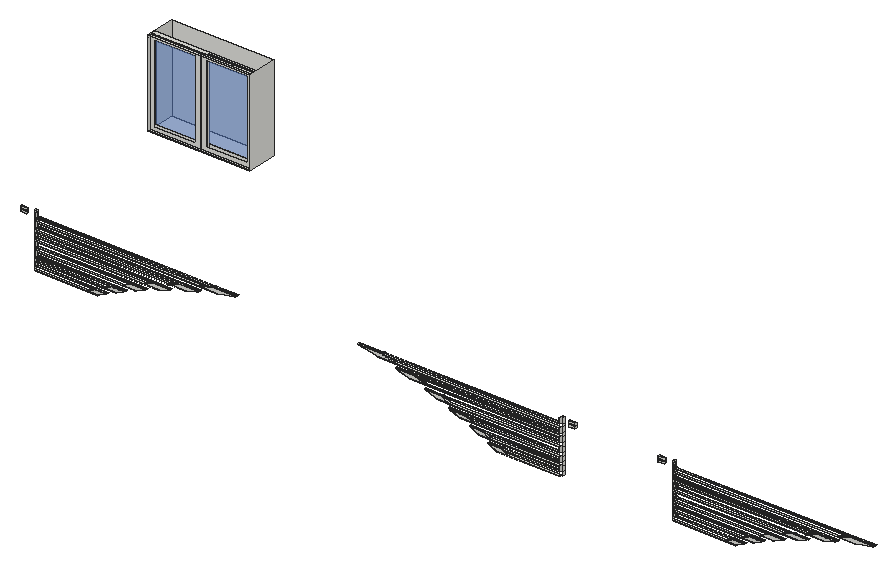
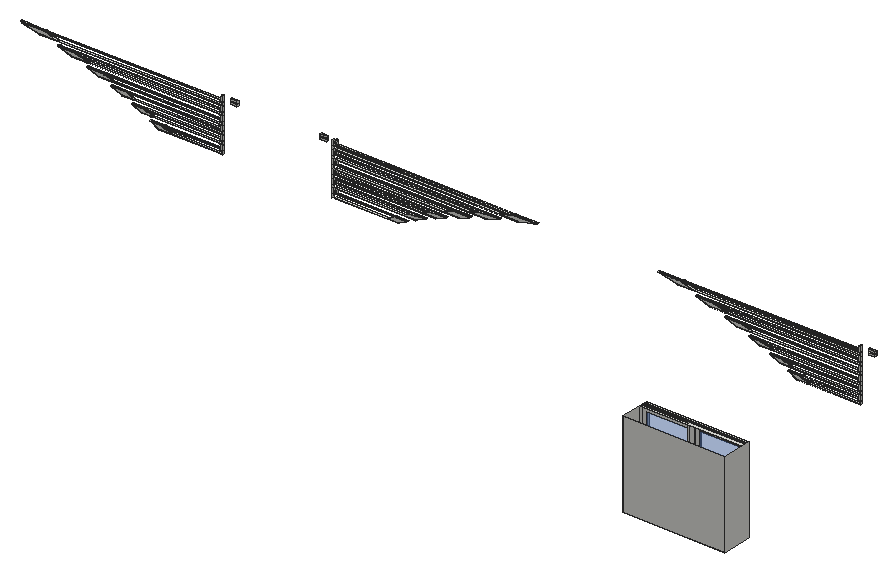
# SketchUp Ruby script. Lengths in inches.
U = 1.inch
M = Sketchup.active_model
def pt(a) = Geom::Point3d.new(a.map { |v| v * U })
def face(e, loops, mat)
  f = e.add_face(loops[0].map { |a| pt(a) })
  loops[1..].each { |l| e.add_face(l.map { |a| pt(a) }).erase! }
  f.material = f.back_material = mat if mat
  f
end
# faces: each face lists its corners as indices into pts; further lists are holes
def faces(e, pts, list, mat = nil) = list.each { |f| face(e, (f[0].is_a?(Array) ? f : [f]).map { |l| l.map { |i| pts[i] } }, mat) }
# xy, xz, yz: faces in a plane at the given z, y or x. An outline is a flat list of corners, or four numbers for a rectangle; further outlines are holes
def ring(l) = l.size == 4 ? [[l[0], l[1]], [l[2], l[1]], [l[2], l[3]], [l[0], l[3]]] : l.each_slice(2).to_a
def flat(e, list, mat, &to3) = list.each { |f| face(e, (f[0].is_a?(Array) ? f : [f]).map { |l| ring(l).map { |u, v| to3.(u, v) } }, mat) }
def xy(e, z, list, mat = nil) = flat(e, list, mat) { |x, y| [x, y, z] }
def xz(e, y, list, mat = nil) = flat(e, list, mat) { |x, z| [x, y, z] }
def yz(e, x, list, mat = nil) = flat(e, list, mat) { |y, z| [x, y, z] }
def lines(e, pts, list) = list.each { |a, b| e.add_line(pt(pts[a]), pt(pts[b])) }
# prism: a flat outline (further loops are holes) pulled along v
def prism(e, loops, v, mat = nil)
  f = face(e, loops, mat); d = Geom::Vector3d.new(v.map { |x| x * U })
  f.pushpull(f.normal.samedirection?(d) ? d.length : -d.length)
end
def box(e, o, s, mat = nil) = prism(e, [[o, [o[0] + s[0], o[1], o[2]], [o[0] + s[0], o[1] + s[1], o[2]], [o[0], o[1] + s[1], o[2]]]], [0, 0, s[2]], mat)
def at(x, y, z, deg = 0) = Geom::Transformation.translation(pt([x, y, z])) * Geom::Transformation.rotation(ORIGIN, Z_AXIS, deg.degrees)
def axes(o, x, y, z) = Geom::Transformation.new([*x, 0, *y, 0, *z, 0, *pt(o).to_a, 1])
def part(name) = M.definitions.add(name)
# library, detail: a bought-in or finely detailed component or shape, given as its bounding box
def library(name, o, s) = part(name).tap { |d| box(d.entities, o, s) }
def detail(e, o, s) = box(e.add_group.entities, o, s)
def put(e, d, t, mat = nil) = e.add_instance(d, t).tap { |i| i.material = mat if mat }
def group(e, t, mat = nil) = e.add_group.tap { |g| g.transformation = t; g.material = mat if mat }.entities
root = M.entities
M.materials.add("[Translucent Glass Blue]").color = [100, 149, 237]
M.materials["[Translucent Glass Blue]"].alpha = 0.5
c1 = part("Janela aluminio")
xy(c1.entities,0,[[0,0,47.24,1.57],[23.62,1.57,47.24,2.76],[0,2.76,25.98,3.9375],[0,3.9375,47.24,5.91]])
xy(c1.entities,43.31,[[0,0,47.24,1.57],[23.62,1.57,47.24,2.76],[0,2.76,0,5.91,47.24,5.91,47.24,3.9375,25.98,3.9375,25.98,2.76],[25.98,2.76,47.24,3.9375]])
xz(c1.entities,1.57,[[0,0,23.62,0,23.62,41.34,21.26,41.34,21.26,1.97,1.97,1.97,1.97,41.34,23.62,41.34,23.62,43.31,0,43.31],[[23.62,0,47.24,43.31],[25.7,1.97,45.28,41.34]]])
xz(c1.entities,2.76,[[[0,0,23.62,43.31],[2.36,2.36,21.26,40.94]],[23.62,0,25.98,43.31]])
xz(c1.entities,2.76,[[2.36,2.36,21.26,40.94]],"[Translucent Glass Blue]")
xz(c1.entities,3.9375,[[25.98,0,25.98,2.36,44.88,2.36,44.88,40.94,25.98,40.94,25.98,43.31,47.24,43.31,47.24,0]])
xz(c1.entities,3.9375,[[25.98,2.36,44.88,40.94]],"[Translucent Glass Blue]")
yz(c1.entities,0,[[0,0,1.57,43.31],[2.76,0,5.91,43.31]])
yz(c1.entities,23.62,[[1.57,0,2.76,43.31]])
yz(c1.entities,25.98,[[2.76,0,3.9375,43.31]])
yz(c1.entities,47.24,[[0,0,1.57,43.31],[1.57,0,2.76,43.31],[3.9375,0,5.91,43.31]])
xy(root,27.6875,[[193.54,12.93,230.17,13.56],[230.17,12.93,237.375,13.56],[518.74,12.93,525.9375,13.56],[525.9375,12.93,562.58,13.56],[643.44,12.93,680.08,13.56],
  [680.08,12.93,687.28,13.56],[193.54,13.81,230.17,14.31],[230.17,13.81,237.375,14.31],[518.74,13.81,525.9375,14.31],[525.9375,13.81,562.58,14.31],
  [643.44,13.81,680.08,14.31],[680.08,13.81,687.28,14.31]])
xy(root,28.18,[[192.75,12.93,230.17,14.31],[230.17,12.93,238.16,14.31],[517.95,12.93,525.9375,14.31],[525.9375,12.93,563.36,14.31],[642.65,12.93,680.08,14.31],
  [680.08,12.93,688.07,14.31]])
xy(root,29.54,[[145.1,172.4375,217.17,193.125]])
xy(root,30.61,[[192.75,12.93,234.88,14.31],[234.88,12.93,242.875,14.31],[513.24,12.93,521.23,14.31],[521.23,12.93,563.36,14.31],[642.65,12.93,684.79,14.31],
  [684.79,12.93,692.78,14.31]])
xy(root,31.1,[[193.54,12.93,234.88,13.56],[234.88,12.93,243.66,13.56],[512.45,12.93,521.23,13.56],[521.23,12.93,562.58,13.56],[643.44,12.93,684.79,13.56],
  [684.79,12.93,693.57,13.56],[193.54,13.81,234.88,14.31],[234.88,13.81,243.66,14.31],[512.45,13.81,521.23,14.31],[521.23,13.81,562.58,14.31],
  [643.44,13.81,684.79,14.31],[684.79,13.81,693.57,14.31]])
xy(root,33.81,[[193.54,12.93,242.07,13.56],[242.07,12.93,249.79,13.56],[506.32,12.93,514.05,13.56],[514.05,12.93,562.58,13.56],[643.44,12.93,691.97,13.56],
  [691.97,12.93,699.7,13.56],[193.54,13.81,242.07,14.31],[242.07,13.81,249.79,14.31],[506.32,13.81,514.05,14.31],[514.05,13.81,562.58,14.31],
  [643.44,13.81,691.97,14.31],[691.97,13.81,699.7,14.31]])
xy(root,34.3,[[192.75,12.93,242.07,14.31],[242.07,12.93,250.58,14.31],[505.53,12.93,514.05,14.31],[514.05,12.93,563.36,14.31],[642.65,12.93,691.97,14.31],
  [691.97,12.93,700.48,14.31]])
xy(root,36.73,[[192.75,12.93,247.27,14.31],[247.27,12.93,255.92,14.31],[500.19,12.93,508.84,14.31],[508.84,12.93,563.36,14.31],[642.65,12.93,697.18,14.31],
  [697.18,12.93,705.83,14.31]])
xy(root,37.22,[[193.54,12.93,247.27,13.56],[247.27,12.93,256.71,13.56],[499.4,12.93,508.84,13.56],[508.84,12.93,562.58,13.56],[643.44,12.93,697.18,13.56],
  [697.18,12.93,706.61,13.56],[193.54,13.81,247.27,14.31],[247.27,13.81,256.71,14.31],[499.4,13.81,508.84,14.31],[508.84,13.81,562.58,14.31],
  [643.44,13.81,697.18,14.31],[697.18,13.81,706.61,14.31]])
xy(root,39.93,[[193.54,12.93,255.42,13.56],[255.42,12.93,263.81,13.56],[492.31,12.93,500.7,13.56],[500.7,12.93,562.58,13.56],[643.44,12.93,705.32,13.56],
  [705.32,12.93,713.71,13.56],[193.54,13.81,255.42,14.31],[255.42,13.81,263.81,14.31],[492.31,13.81,500.7,14.31],[500.7,13.81,562.58,14.31],
  [643.44,13.81,705.32,14.31],[705.32,13.81,713.71,14.31]])
xy(root,40.42,[[192.75,12.93,255.42,14.31],[255.42,12.93,264.59,14.31],[491.52,12.93,500.7,14.31],[500.7,12.93,563.36,14.31],[642.65,12.93,705.32,14.31],
  [705.32,12.93,714.5,14.31]])
xy(root,42.85,[[192.75,12.93,261.22,14.31],[261.22,12.93,270.68,14.31],[485.43,12.93,494.89,14.31],[494.89,12.93,563.36,14.31],[642.65,12.93,711.13,14.31],
  [711.13,12.93,720.59,14.31]])
xy(root,43.34,[[193.54,12.93,261.22,13.56],[261.22,12.93,271.47,13.56],[484.64,12.93,494.89,13.56],[494.89,12.93,562.58,13.56],[643.44,12.93,711.13,13.56],
  [711.13,12.93,721.38,13.56],[193.54,13.81,261.22,14.31],[261.22,13.81,271.47,14.31],[484.64,13.81,494.89,14.31],[494.89,13.81,562.58,14.31],
  [643.44,13.81,711.13,14.31],[711.13,13.81,721.38,14.31]])
xy(root,46.05,[[193.54,12.93,270.51,13.56],[270.51,12.93,279.92,13.56],[476.19,12.93,485.61,13.56],[485.61,12.93,562.58,13.56],[643.44,12.93,720.41,13.56],
  [720.41,12.93,729.83,13.56],[193.54,13.81,270.51,14.31],[270.51,13.81,279.92,14.31],[476.19,13.81,485.61,14.31],[485.61,13.81,562.58,14.31],
  [643.44,13.81,720.41,14.31],[720.41,13.81,729.83,14.31]])
xy(root,46.54,[[192.75,12.93,270.51,14.31],[270.51,12.93,280.71,14.31],[475.4,12.93,485.61,14.31],[485.61,12.93,563.36,14.31],[642.65,12.93,720.41,14.31],
  [720.41,12.93,730.62,14.31]])
xy(root,48.97,[[192.75,12.93,277.22,14.31],[277.22,12.93,287.71,14.31],[468.41,12.93,478.89,14.31],[478.89,12.93,563.36,14.31],[642.65,12.93,727.13,14.31],
  [727.13,12.93,737.61,14.31]])
xy(root,49.46,[[193.54,12.93,277.22,13.56],[277.22,12.93,288.49,13.56],[467.62,12.93,478.89,13.56],[478.89,12.93,562.58,13.56],[643.44,12.93,727.13,13.56],
  [727.13,12.93,738.4,13.56],[193.54,13.81,277.22,14.31],[277.22,13.81,288.49,14.31],[467.62,13.81,478.89,14.31],[478.89,13.81,562.58,14.31],
  [643.44,13.81,727.13,14.31],[727.13,13.81,738.4,14.31]])
xy(root,52.17,[[193.54,12.93,287.89,13.56],[287.89,12.93,298.9,13.56],[457.21,12.93,468.22,13.56],[468.22,12.93,562.58,13.56],[643.44,12.93,737.8,13.56],
  [737.8,12.93,748.81,13.56],[193.54,13.81,287.89,14.31],[287.89,13.81,298.9,14.31],[457.21,13.81,468.22,14.31],[468.22,13.81,562.58,14.31],
  [643.44,13.81,737.8,14.31],[737.8,13.81,748.81,14.31]])
xy(root,52.67,[[192.75,12.93,287.89,14.31],[287.89,12.93,299.6875,14.31],[456.42,12.93,468.22,14.31],[468.22,12.93,563.36,14.31],[642.65,12.93,737.8,14.31],
  [737.8,12.93,749.6,14.31]])
xy(root,55.09,[[192.75,12.93,296.02,14.31],[296.02,12.93,308.16,14.31],[447.95,12.93,460.1,14.31],[460.1,12.93,563.36,14.31],[642.65,12.93,745.92,14.31],
  [745.92,12.93,758.07,14.31]])
xy(root,55.59,[[193.54,12.93,296.02,13.56],[296.02,12.93,308.95,13.56],[447.17,12.93,460.1,13.56],[460.1,12.93,562.58,13.56],[643.44,12.93,745.92,13.56],
  [745.92,12.93,758.85,13.56],[193.54,13.81,296.02,14.31],[296.02,13.81,308.95,14.31],[447.17,13.81,460.1,14.31],[460.1,13.81,562.58,14.31],
  [643.44,13.81,745.92,14.31],[745.92,13.81,758.85,14.31]])
xy(root,58.29,[[193.54,12.93,309.22,13.56],[309.22,12.93,321.26,13.56],[434.85,12.93,446.9,13.56],[446.9,12.93,562.58,13.56],[643.44,12.93,759.12,13.56],
  [759.12,12.93,771.16,13.56],[193.54,13.81,309.22,14.31],[309.22,13.81,321.26,14.31],[434.85,13.81,446.9,14.31],[446.9,13.81,562.58,14.31],
  [643.44,13.81,759.12,14.31],[759.12,13.81,771.16,14.31]])
xy(root,58.79,[[192.75,12.93,309.22,14.31],[446.9,12.93,563.36,14.31],[642.65,12.93,759.12,14.31]])
xy(root,61.21,[[192.75,12.93,318.8,14.31],[318.8,12.93,334.49,14.31],[421.62,12.93,437.31,14.31],[437.31,12.93,563.36,14.31],[642.65,12.93,768.71,14.31],
  [768.71,12.93,784.4,14.31]])
xy(root,61.46,[[182.38,13.24,186.86,14.43],[569.26,13.24,573.73,14.43],[632.29,13.24,636.76,14.43]])
xy(root,61.71,[[193.54,12.93,318.8,13.56],[318.8,12.93,335.28,13.56],[420.83,12.93,437.31,13.56],[437.31,12.93,562.58,13.56],[643.44,12.93,768.71,13.56],
  [768.71,12.93,785.19,13.56],[193.54,13.81,318.8,14.31],[318.8,13.81,335.28,14.31],[420.83,13.81,437.31,14.31],[437.31,13.81,562.58,14.31],
  [643.44,13.81,768.71,14.31],[768.71,13.81,785.19,14.31]])
xy(root,62.75,[[182.38,13.24,186.86,14.43],[569.26,13.24,573.73,14.43],[632.29,13.24,636.76,14.43]])
xy(root,63.67,[[182.38,13.24,186.86,14.43],[569.26,13.24,573.73,14.43],[632.29,13.24,636.76,14.43]])
xz(root,12.93,[[230.17,28.18,238.16,28.18,242.875,30.61,234.88,30.61],[517.95,28.18,513.24,30.61,521.23,30.61,525.9375,28.18],[680.08,28.18,688.07,28.18,692.78,30.61,684.79,30.61],[242.07,34.3,250.58,34.3,255.92,36.73,247.27,36.73,243.08,34.82],[505.53,34.3,500.19,36.73,508.84,36.73,513.03,34.82,514.05,34.3],
  [691.97,34.3,700.48,34.3,705.83,36.73,697.18,36.73,692.98,34.82],[255.42,40.42,264.59,40.42,270.68,42.85,261.22,42.85,257.42,41.34],[491.52,40.42,485.43,42.85,494.89,42.85,498.6875,41.34,500.7,40.42],[705.32,40.42,714.5,40.42,720.59,42.85,711.13,42.85,707.33,41.34],[270.51,46.54,280.71,46.54,287.71,48.97,277.22,48.97,272.375,47.29],
  [475.4,46.54,468.41,48.97,478.89,48.97,483.74,47.29,485.61,46.54],[720.41,46.54,730.62,46.54,737.61,48.97,727.13,48.97,722.28,47.29],[287.89,52.67,299.6875,52.67,305.91,54.52,308.16,55.09,296.02,55.09],[456.42,52.67,450.21,54.52,447.95,55.09,460.1,55.09,468.22,52.67],[737.8,52.67,749.6,52.67,755.8125,54.52,758.07,55.09,745.92,55.09],
  [322.05,58.6,322.92,58.79,334.49,61.21,318.8,61.21,309.22,58.79,322.05,58.79],[434.07,58.6,433.19,58.79,421.62,61.21,437.31,61.21,446.9,58.79,434.07,58.79],[771.95,58.6,772.83,58.79,784.4,61.21,768.71,61.21,759.12,58.79,771.95,58.79]])
xz(root,13.24,[[182.38,61.46,186.86,62.75],[569.26,61.46,573.73,62.75],[632.29,61.46,636.76,62.75],[182.38,63.67,186.86,64.96],[569.26,63.67,573.73,64.96],
  [632.29,63.67,636.76,64.96]])
xz(root,14.31,[[230.17,28.18,234.88,30.61,242.875,30.61,238.16,28.18],[517.95,28.18,525.9375,28.18,521.23,30.61,513.24,30.61],[680.08,28.18,684.79,30.61,692.78,30.61,688.07,28.18],[242.07,34.3,243.08,34.82,247.27,36.73,255.92,36.73,250.58,34.3],[505.53,34.3,514.05,34.3,513.03,34.82,508.84,36.73,500.19,36.73],
  [691.97,34.3,692.98,34.82,697.18,36.73,705.83,36.73,700.48,34.3],[255.42,40.42,257.42,41.34,261.22,42.85,270.68,42.85,264.59,40.42],[491.52,40.42,500.7,40.42,498.6875,41.34,494.89,42.85,485.43,42.85],[705.32,40.42,707.33,41.34,711.13,42.85,720.59,42.85,714.5,40.42],[270.51,46.54,272.375,47.29,277.22,48.97,287.71,48.97,280.71,46.54],
  [475.4,46.54,485.61,46.54,483.74,47.29,478.89,48.97,468.41,48.97],[720.41,46.54,722.28,47.29,727.13,48.97,737.61,48.97,730.62,46.54],[287.89,52.67,296.02,55.09,308.16,55.09,305.91,54.52,299.6875,52.67],[456.42,52.67,468.22,52.67,460.1,55.09,447.95,55.09,450.21,54.52],[737.8,52.67,745.92,55.09,758.07,55.09,755.8125,54.52,749.6,52.67],
  [322.05,58.6,322.05,58.79,309.22,58.79,318.8,61.21,334.49,61.21,322.92,58.79],[434.07,58.6,434.07,58.79,446.9,58.79,437.31,61.21,421.62,61.21,433.19,58.79],[771.95,58.6,771.95,58.79,759.12,58.79,768.71,61.21,784.4,61.21,772.83,58.79]])
xz(root,14.43,[[182.38,61.46,186.86,62.75],[569.26,61.46,573.73,62.75],[632.29,61.46,636.76,62.75],[182.38,63.67,186.86,64.96],[569.26,63.67,573.73,64.96],
  [632.29,63.67,636.76,64.96]])
xz(root,193.125,[[145.1,29.54,217.17,90.15]])
yz(root,145.1,[[172.4375,29.54,193.125,90.15]])
yz(root,182.38,[[13.24,61.46,14.43,62.75],[13.24,63.67,14.43,64.96]])
yz(root,191.63,[[14.12,28.18,15.56,30.61],[14.12,30.61,15.56,34.3],[14.12,34.3,15.56,36.73],[14.12,36.73,15.56,40.42],[14.12,40.42,15.56,42.85],
  [14.12,42.85,15.56,46.54],[14.12,46.54,15.56,48.97],[14.12,48.97,15.56,52.67],[14.12,52.67,15.56,55.09],[14.12,55.09,15.56,58.79],
  [14.12,58.79,15.56,61.21],[14.12,61.21,15.56,64.91]])
yz(root,192.75,[[12.93,30.61,14.31,34.3],[14.31,30.61,15.56,34.3],[12.93,36.73,14.31,40.42],[14.31,36.73,15.56,40.42],[12.93,42.85,14.31,46.54],
  [14.31,42.85,15.56,46.54],[12.93,48.97,14.31,52.67],[14.31,48.97,15.56,52.67],[12.93,55.09,14.31,58.79],[14.31,55.09,15.56,58.79],
  [12.93,61.21,14.31,64.91],[14.31,61.21,15.56,64.91]])
yz(root,193.54,[[12.93,31.1,13.56,33.81],[13.81,31.1,14.31,33.81],[12.93,37.22,13.56,39.93],[13.81,37.22,14.31,39.93],[12.93,43.34,13.56,46.05],
  [13.81,43.34,14.31,46.05],[12.93,49.46,13.56,52.17],[13.81,49.46,14.31,52.17],[12.93,55.59,13.56,58.29],[13.81,55.59,14.31,58.29],
  [12.93,61.71,13.56,64.41],[13.81,61.71,14.31,64.41]])
yz(root,217.17,[[172.4375,29.54,193.125,90.15]])
yz(root,562.58,[[12.93,31.1,13.56,33.81],[13.81,31.1,14.31,33.81],[12.93,37.22,13.56,39.93],[13.81,37.22,14.31,39.93],[12.93,43.34,13.56,46.05],
  [13.81,43.34,14.31,46.05],[12.93,49.46,13.56,52.17],[13.81,49.46,14.31,52.17],[12.93,55.59,13.56,58.29],[13.81,55.59,14.31,58.29],
  [12.93,61.71,13.56,64.41],[13.81,61.71,14.31,64.41]])
yz(root,563.36,[[12.93,30.61,14.31,34.3],[14.31,30.61,15.56,34.3],[12.93,36.73,14.31,40.42],[14.31,36.73,15.56,40.42],[12.93,42.85,14.31,46.54],
  [14.31,42.85,15.56,46.54],[12.93,48.97,14.31,52.67],[14.31,48.97,15.56,52.67],[12.93,55.09,14.31,58.79],[14.31,55.09,15.56,58.79],
  [12.93,61.21,14.31,64.91],[14.31,61.21,15.56,64.91]])
yz(root,564.48,[[14.12,28.18,15.56,30.61],[14.12,30.61,15.56,34.3],[14.12,34.3,15.56,36.73],[14.12,36.73,15.56,40.42],[14.12,40.42,15.56,42.85],
  [14.12,42.85,15.56,46.54],[14.12,46.54,15.56,48.97],[14.12,48.97,15.56,52.67],[14.12,52.67,15.56,55.09],[14.12,55.09,15.56,58.79],
  [14.12,58.79,15.56,61.21],[14.12,61.21,15.56,64.91]])
yz(root,573.73,[[13.24,61.46,14.43,62.75],[13.24,63.67,14.43,64.96]])
yz(root,632.29,[[13.24,61.46,14.43,62.75],[13.24,63.67,14.43,64.96]])
yz(root,641.54,[[14.12,28.18,15.56,30.61],[14.12,30.61,15.56,34.3],[14.12,34.3,15.56,36.73],[14.12,36.73,15.56,40.42],[14.12,40.42,15.56,42.85],
  [14.12,42.85,15.56,46.54],[14.12,46.54,15.56,48.97],[14.12,48.97,15.56,52.67],[14.12,52.67,15.56,55.09],[14.12,55.09,15.56,58.79],
  [14.12,58.79,15.56,61.21],[14.12,61.21,15.56,64.91]])
yz(root,642.65,[[12.93,30.61,14.31,34.3],[14.31,30.61,15.56,34.3],[12.93,36.73,14.31,40.42],[14.31,36.73,15.56,40.42],[12.93,42.85,14.31,46.54],
  [14.31,42.85,15.56,46.54],[12.93,48.97,14.31,52.67],[14.31,48.97,15.56,52.67],[12.93,55.09,14.31,58.79],[14.31,55.09,15.56,58.79],
  [12.93,61.21,14.31,64.91],[14.31,61.21,15.56,64.91]])
yz(root,643.44,[[12.93,31.1,13.56,33.81],[13.81,31.1,14.31,33.81],[12.93,37.22,13.56,39.93],[13.81,37.22,14.31,39.93],[12.93,43.34,13.56,46.05],
  [13.81,43.34,14.31,46.05],[12.93,49.46,13.56,52.17],[13.81,49.46,14.31,52.17],[12.93,55.59,13.56,58.29],[13.81,55.59,14.31,58.29],
  [12.93,61.71,13.56,64.41],[13.81,61.71,14.31,64.41]])
p = [[234.88,14.31,30.61],[230.17,14.31,28.18],[230.17,12.93,28.18],[234.88,12.93,30.61],[238.16,14.31,28.18],[242.875,14.31,30.61],
  [242.875,12.93,30.61],[238.16,12.93,28.18],[517.95,14.31,28.18],[513.24,14.31,30.61],[513.24,12.93,30.61],[517.95,12.93,28.18],
  [521.23,14.31,30.61],[525.9375,14.31,28.18],[525.9375,12.93,28.18],[521.23,12.93,30.61],[684.79,14.31,30.61],[680.08,14.31,28.18],
  [680.08,12.93,28.18],[684.79,12.93,30.61],[688.07,14.31,28.18],[692.78,14.31,30.61],[692.78,12.93,30.61],[688.07,12.93,28.18],
  [243.08,14.31,34.82],[242.07,14.31,34.3],[242.07,12.93,34.3],[243.08,12.93,34.82],[250.58,14.31,34.3],[255.92,14.31,36.73],
  [255.92,12.93,36.73],[250.58,12.93,34.3],[505.53,14.31,34.3],[500.19,14.31,36.73],[500.19,12.93,36.73],[505.53,12.93,34.3],
  [513.03,14.31,34.82],[514.05,14.31,34.3],[514.05,12.93,34.3],[513.03,12.93,34.82],[692.98,14.31,34.82],[691.97,14.31,34.3],
  [691.97,12.93,34.3],[692.98,12.93,34.82],[700.48,14.31,34.3],[705.83,14.31,36.73],[705.83,12.93,36.73],[700.48,12.93,34.3],
  [247.27,14.31,36.73],[247.27,12.93,36.73],[508.84,14.31,36.73],[508.84,12.93,36.73],[697.18,14.31,36.73],[697.18,12.93,36.73],
  [257.42,14.31,41.34],[255.42,14.31,40.42],[255.42,12.93,40.42],[257.42,12.93,41.34],[264.59,14.31,40.42],[270.68,14.31,42.85],
  [270.68,12.93,42.85],[264.59,12.93,40.42],[491.52,14.31,40.42],[485.43,14.31,42.85],[485.43,12.93,42.85],[491.52,12.93,40.42],
  [498.6875,14.31,41.34],[500.7,14.31,40.42],[500.7,12.93,40.42],[498.6875,12.93,41.34],[707.33,14.31,41.34],[705.32,14.31,40.42],
  [705.32,12.93,40.42],[707.33,12.93,41.34],[714.5,14.31,40.42],[720.59,14.31,42.85],[720.59,12.93,42.85],[714.5,12.93,40.42],
  [261.22,14.31,42.85],[261.22,12.93,42.85],[494.89,14.31,42.85],[494.89,12.93,42.85],[711.13,14.31,42.85],[711.13,12.93,42.85],
  [272.375,14.31,47.29],[270.51,14.31,46.54],[270.51,12.93,46.54],[272.375,12.93,47.29],[280.71,14.31,46.54],[287.71,14.31,48.97],
  [287.71,12.93,48.97],[280.71,12.93,46.54],[475.4,14.31,46.54],[468.41,14.31,48.97],[468.41,12.93,48.97],[475.4,12.93,46.54],
  [483.74,14.31,47.29],[485.61,14.31,46.54],[485.61,12.93,46.54],[483.74,12.93,47.29],[722.28,14.31,47.29],[720.41,14.31,46.54],
  [720.41,12.93,46.54],[722.28,12.93,47.29],[730.62,14.31,46.54],[737.61,14.31,48.97],[737.61,12.93,48.97],[730.62,12.93,46.54],
  [277.22,14.31,48.97],[277.22,12.93,48.97],[478.89,14.31,48.97],[478.89,12.93,48.97],[727.13,14.31,48.97],[727.13,12.93,48.97],
  [296.02,14.31,55.09],[287.89,14.31,52.67],[287.89,12.93,52.67],[296.02,12.93,55.09],[299.6875,14.31,52.67],[305.91,14.31,54.52],
  [305.91,12.93,54.52],[299.6875,12.93,52.67],[456.42,14.31,52.67],[450.21,14.31,54.52],[450.21,12.93,54.52],[456.42,12.93,52.67],
  [460.1,14.31,55.09],[468.22,14.31,52.67],[468.22,12.93,52.67],[460.1,12.93,55.09],[745.92,14.31,55.09],[737.8,14.31,52.67],
  [737.8,12.93,52.67],[745.92,12.93,55.09],[749.6,14.31,52.67],[755.8125,14.31,54.52],[755.8125,12.93,54.52],[749.6,12.93,52.67],
  [308.16,14.31,55.09],[308.16,12.93,55.09],[447.95,14.31,55.09],[447.95,12.93,55.09],[758.07,14.31,55.09],[758.07,12.93,55.09],
  [322.05,14.31,58.6],[322.92,14.31,58.79],[334.49,14.31,61.21],[334.49,12.93,61.21],[322.92,12.93,58.79],[322.05,12.93,58.6],
  [434.07,14.31,58.6],[433.19,14.31,58.79],[421.62,14.31,61.21],[421.62,12.93,61.21],[433.19,12.93,58.79],[434.07,12.93,58.6],
  [771.95,14.31,58.6],[772.83,14.31,58.79],[784.4,14.31,61.21],[784.4,12.93,61.21],[772.83,12.93,58.79],[771.95,12.93,58.6],
  [318.8,14.31,61.21],[309.22,14.31,58.79],[309.22,12.93,58.79],[318.8,12.93,61.21],[437.31,14.31,61.21],[446.9,14.31,58.79],
  [446.9,12.93,58.79],[437.31,12.93,61.21],[768.71,14.31,61.21],[759.12,14.31,58.79],[759.12,12.93,58.79],[768.71,12.93,61.21]]
faces(root,p,[[0,1,2,3],[4,5,6,7],[8,9,10,11],[12,13,14,15],[16,17,18,19],[20,21,22,23],[24,25,26,27],[28,29,30,31],
  [32,33,34,35],[36,37,38,39],[40,41,42,43],[44,45,46,47],[48,24,27,49],[50,36,39,51],[52,40,43,53],[54,55,56,57],
  [58,59,60,61],[62,63,64,65],[66,67,68,69],[70,71,72,73],[74,75,76,77],[78,54,57,79],[80,66,69,81],[82,70,73,83],
  [84,85,86,87],[88,89,90,91],[92,93,94,95],[96,97,98,99],[100,101,102,103],[104,105,106,107],[108,84,87,109],[110,96,99,111],
  [112,100,103,113],[114,115,116,117],[118,119,120,121],[122,123,124,125],[126,127,128,129],[130,131,132,133],[134,135,136,137],[119,138,139,120],
  [123,140,141,124],[135,142,143,136],[144,145,146,147,148,149],[150,151,152,153,154,155],[156,157,158,159,160,161],[162,163,164,165],[166,167,168,169],[170,171,172,173]])
put(root,c1,axes([145.1,172.4375,29.69],[1.5254,0,0],[0,1,0],[0,0,1.39595]))
